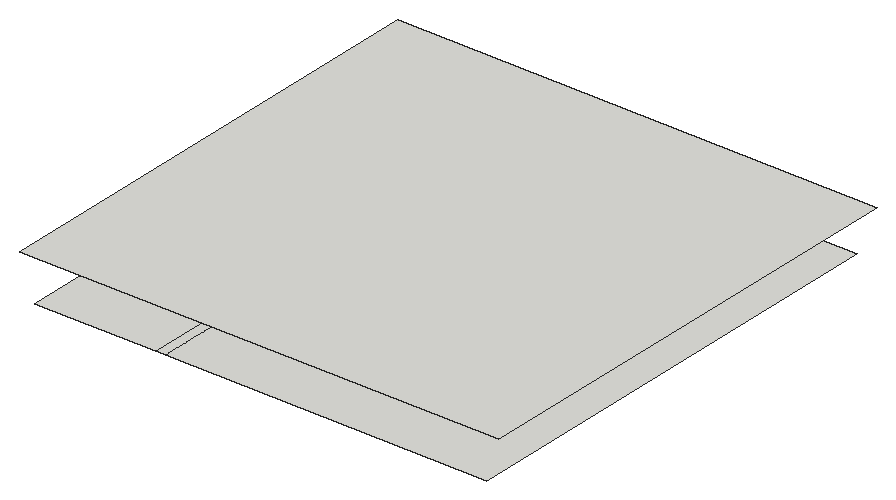
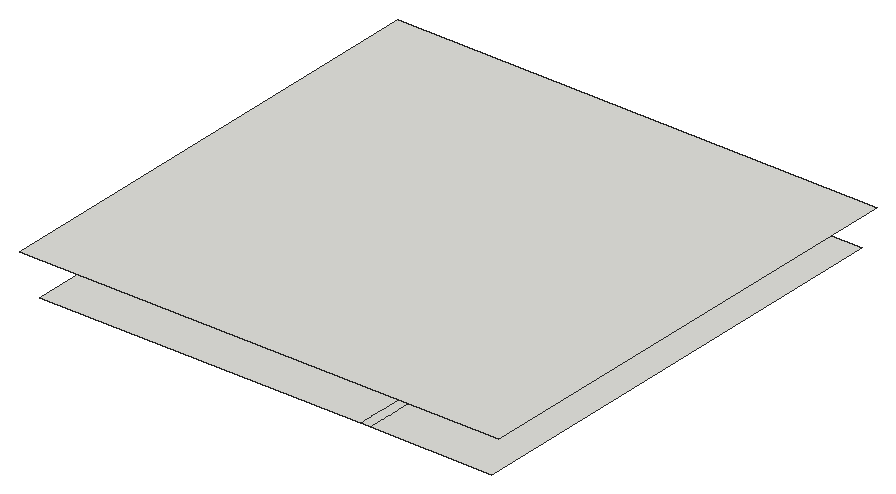
# SketchUp Ruby script. Lengths in inches.
U = 1.inch
M = Sketchup.active_model
def pt(a) = Geom::Point3d.new(a.map { |v| v * U })
def face(e, loops, mat)
  f = e.add_face(loops[0].map { |a| pt(a) })
  loops[1..].each { |l| e.add_face(l.map { |a| pt(a) }).erase! }
  f.material = f.back_material = mat if mat
  f
end
# faces: each face lists its corners as indices into pts; further lists are holes
def faces(e, pts, list, mat = nil) = list.each { |f| face(e, (f[0].is_a?(Array) ? f : [f]).map { |l| l.map { |i| pts[i] } }, mat) }
# xy, xz, yz: faces in a plane at the given z, y or x. An outline is a flat list of corners, or four numbers for a rectangle; further outlines are holes
def ring(l) = l.size == 4 ? [[l[0], l[1]], [l[2], l[1]], [l[2], l[3]], [l[0], l[3]]] : l.each_slice(2).to_a
def flat(e, list, mat, &to3) = list.each { |f| face(e, (f[0].is_a?(Array) ? f : [f]).map { |l| ring(l).map { |u, v| to3.(u, v) } }, mat) }
def xy(e, z, list, mat = nil) = flat(e, list, mat) { |x, y| [x, y, z] }
def xz(e, y, list, mat = nil) = flat(e, list, mat) { |x, z| [x, y, z] }
def yz(e, x, list, mat = nil) = flat(e, list, mat) { |y, z| [x, y, z] }
def lines(e, pts, list) = list.each { |a, b| e.add_line(pt(pts[a]), pt(pts[b])) }
# prism: a flat outline (further loops are holes) pulled along v
def prism(e, loops, v, mat = nil)
  f = face(e, loops, mat); d = Geom::Vector3d.new(v.map { |x| x * U })
  f.pushpull(f.normal.samedirection?(d) ? d.length : -d.length)
end
def box(e, o, s, mat = nil) = prism(e, [[o, [o[0] + s[0], o[1], o[2]], [o[0] + s[0], o[1] + s[1], o[2]], [o[0], o[1] + s[1], o[2]]]], [0, 0, s[2]], mat)
def at(x, y, z, deg = 0) = Geom::Transformation.translation(pt([x, y, z])) * Geom::Transformation.rotation(ORIGIN, Z_AXIS, deg.degrees)
def axes(o, x, y, z) = Geom::Transformation.new([*x, 0, *y, 0, *z, 0, *pt(o).to_a, 1])
def part(name) = M.definitions.add(name)
# library, detail: a bought-in or finely detailed component or shape, given as its bounding box
def library(name, o, s) = part(name).tap { |d| box(d.entities, o, s) }
def detail(e, o, s) = box(e.add_group.entities, o, s)
def put(e, d, t, mat = nil) = e.add_instance(d, t).tap { |i| i.material = mat if mat }
def group(e, t, mat = nil) = e.add_group.tap { |g| g.transformation = t; g.material = mat if mat }.entities
root = M.entities
M.materials.add("[Wood Veneer 01]").color = [120, 70, 37]
xy(root,152.95,[[[101.27,14.42,137.48,92.99],[119.24,38.31,120.375,38.46,121.43,38.89,122.33,39.59,123.03,40.5,123.47,41.55,123.62,42.68,123.47,43.82,123.03,44.87,122.33,45.78,121.43,46.47,120.375,46.91,119.24,47.06,118.11,46.91,117.05,46.47,116.15,45.78,115.45,44.87,115.02,43.82,114.87,42.68,115.02,41.55,115.45,40.5,116.15,39.59,117.05,38.89,118.11,38.46]],[[144.99,14.42,181.2,92.99],[162.74,38.31,163.875,38.46,164.93,38.89,165.83,39.59,166.53,40.5,166.97,41.55,167.12,42.68,166.97,43.82,166.53,44.87,165.83,45.78,164.93,46.47,163.875,46.91,162.74,47.06,161.61,46.91,160.55,46.47,159.65,45.78,158.95,44.87,158.52,43.82,158.37,42.68,158.52,41.55,158.95,40.5,159.65,39.59,160.55,38.89,161.61,38.46]],[[188.72,14.42,224.93,92.99],[207.49,38.31,208.625,38.46,209.68,38.89,210.58,39.59,211.28,40.5,211.72,41.55,211.87,42.68,211.72,43.82,211.28,44.87,210.58,45.78,209.68,46.47,208.625,46.91,207.49,47.06,206.36,46.91,205.3,46.47,204.4,45.78,203.7,44.87,203.27,43.82,203.12,42.68,203.27,41.55,203.7,40.5,204.4,39.59,205.3,38.89,206.36,38.46]],[[232.44,14.42,268.65,92.99],[253.24,38.31,254.375,38.46,255.43,38.89,256.33,39.59,257.03,40.5,257.47,41.55,257.62,42.68,257.47,43.82,257.03,44.87,256.33,45.78,255.43,46.47,254.375,46.91,253.24,47.06,252.11,46.91,251.05,46.47,250.15,45.78,249.45,44.87,249.02,43.82,248.87,42.68,249.02,41.55,249.45,40.5,250.15,39.59,251.05,38.89,252.11,38.46]],[144.74,96.75,226.06,182.83],
  [[101.27,100.5,137.48,179.07],[119.24,133.62,120.375,133.77,121.43,134.21,122.33,134.9,123.03,135.81,123.47,136.86,123.62,138,123.47,139.13,123.03,140.18,122.33,141.09,121.43,141.78,120.375,142.22,119.24,142.37,118.11,142.22,117.05,141.78,116.15,141.09,115.45,140.18,115.02,139.13,114.87,138,115.02,136.86,115.45,135.81,116.15,134.9,117.05,134.21,118.11,133.77]],[[232.44,100.5,268.65,179.07],[250.49,133.62,251.625,133.77,252.68,134.21,253.58,134.9,254.28,135.81,254.72,136.86,254.87,138,254.72,139.13,254.28,140.18,253.58,141.09,252.68,141.78,251.625,142.22,250.49,142.37,249.36,142.22,248.3,141.78,247.4,141.09,246.7,140.18,246.27,139.13,246.12,138,246.27,136.86,246.7,135.81,247.4,134.9,248.3,134.21,249.36,133.77]],[[101.27,186.58,137.48,265.15],[117.68,218.37,118.8125,218.52,119.87,218.96,120.77,219.65,121.47,220.56,121.9,221.61,122.05,222.75,121.9,223.88,121.47,224.93,120.77,225.84,119.87,226.53,118.8125,226.97,117.68,227.12,116.55,226.97,115.49,226.53,114.59,225.84,113.89,224.93,113.45,223.88,113.3,222.75,113.45,221.61,113.89,220.56,114.59,219.65,115.49,218.96,116.55,218.52]],[[144.99,186.58,181.2,265.15],[162.87,218.37,164,218.52,165.05,218.96,165.96,219.65,166.66,220.56,167.09,221.61,167.24,222.75,167.09,223.88,166.66,224.93,165.96,225.84,165.05,226.53,164,226.97,162.87,227.12,161.73,226.97,160.68,226.53,159.77,225.84,159.08,224.93,158.64,223.88,158.49,222.75,158.64,221.61,159.08,220.56,159.77,219.65,160.68,218.96,161.73,218.52]],[[188.72,186.58,224.93,265.15],[204.43,218.37,205.5625,218.52,206.62,218.96,207.52,219.65,208.22,220.56,208.65,221.61,208.8,222.75,208.65,223.88,208.22,224.93,207.52,225.84,206.62,226.53,205.5625,226.97,204.43,227.12,203.3,226.97,202.24,226.53,201.34,225.84,200.64,224.93,200.2,223.88,200.05,222.75,200.2,221.61,200.64,220.56,201.34,219.65,202.24,218.96,203.3,218.52]],
  [[232.44,186.58,268.65,265.15],[250.49,218.37,251.625,218.52,252.68,218.96,253.58,219.65,254.28,220.56,254.72,221.61,254.87,222.75,254.72,223.88,254.28,224.93,253.58,225.84,252.68,226.53,251.625,226.97,250.49,227.12,249.36,226.97,248.3,226.53,247.4,225.84,246.7,224.93,246.27,223.88,246.12,222.75,246.27,221.61,246.7,220.56,247.4,219.65,248.3,218.96,249.36,218.52]]],"[Wood Veneer 01]")
xy(root,154.7,[[119.24,38.31,118.11,38.46,117.05,38.89,116.15,39.59,115.45,40.5,115.02,41.55,114.87,42.68,115.02,43.82,115.45,44.87,116.15,45.78,117.05,46.47,118.11,46.91,119.24,47.06,120.375,46.91,121.43,46.47,122.33,45.78,123.03,44.87,123.47,43.82,123.62,42.68,123.47,41.55,123.03,40.5,122.33,39.59,121.43,38.89,120.375,38.46],[162.74,38.31,161.61,38.46,160.55,38.89,159.65,39.59,158.95,40.5,158.52,41.55,158.37,42.68,158.52,43.82,158.95,44.87,159.65,45.78,160.55,46.47,161.61,46.91,162.74,47.06,163.875,46.91,164.93,46.47,165.83,45.78,166.53,44.87,166.97,43.82,167.12,42.68,166.97,41.55,166.53,40.5,165.83,39.59,164.93,38.89,163.875,38.46],[207.49,38.31,206.36,38.46,205.3,38.89,204.4,39.59,203.7,40.5,203.27,41.55,203.12,42.68,203.27,43.82,203.7,44.87,204.4,45.78,205.3,46.47,206.36,46.91,207.49,47.06,208.625,46.91,209.68,46.47,210.58,45.78,211.28,44.87,211.72,43.82,211.87,42.68,211.72,41.55,211.28,40.5,210.58,39.59,209.68,38.89,208.625,38.46],[253.24,38.31,252.11,38.46,251.05,38.89,250.15,39.59,249.45,40.5,249.02,41.55,248.87,42.68,249.02,43.82,249.45,44.87,250.15,45.78,251.05,46.47,252.11,46.91,253.24,47.06,254.375,46.91,255.43,46.47,256.33,45.78,257.03,44.87,257.47,43.82,257.62,42.68,257.47,41.55,257.03,40.5,256.33,39.59,255.43,38.89,254.375,38.46],[119.24,133.62,118.11,133.77,117.05,134.21,116.15,134.9,115.45,135.81,115.02,136.86,114.87,138,115.02,139.13,115.45,140.18,116.15,141.09,117.05,141.78,118.11,142.22,119.24,142.37,120.375,142.22,121.43,141.78,122.33,141.09,123.03,140.18,123.47,139.13,123.62,138,123.47,136.86,123.03,135.81,122.33,134.9,121.43,134.21,120.375,133.77],
  [250.49,133.62,249.36,133.77,248.3,134.21,247.4,134.9,246.7,135.81,246.27,136.86,246.12,138,246.27,139.13,246.7,140.18,247.4,141.09,248.3,141.78,249.36,142.22,250.49,142.37,251.625,142.22,252.68,141.78,253.58,141.09,254.28,140.18,254.72,139.13,254.87,138,254.72,136.86,254.28,135.81,253.58,134.9,252.68,134.21,251.625,133.77],[117.68,218.37,116.55,218.52,115.49,218.96,114.59,219.65,113.89,220.56,113.45,221.61,113.3,222.75,113.45,223.88,113.89,224.93,114.59,225.84,115.49,226.53,116.55,226.97,117.68,227.12,118.8125,226.97,119.87,226.53,120.77,225.84,121.47,224.93,121.9,223.88,122.05,222.75,121.9,221.61,121.47,220.56,120.77,219.65,119.87,218.96,118.8125,218.52],[162.87,218.37,161.73,218.52,160.68,218.96,159.77,219.65,159.08,220.56,158.64,221.61,158.49,222.75,158.64,223.88,159.08,224.93,159.77,225.84,160.68,226.53,161.73,226.97,162.87,227.12,164,226.97,165.05,226.53,165.96,225.84,166.66,224.93,167.09,223.88,167.24,222.75,167.09,221.61,166.66,220.56,165.96,219.65,165.05,218.96,164,218.52],[204.43,218.37,203.3,218.52,202.24,218.96,201.34,219.65,200.64,220.56,200.2,221.61,200.05,222.75,200.2,223.88,200.64,224.93,201.34,225.84,202.24,226.53,203.3,226.97,204.43,227.12,205.5625,226.97,206.62,226.53,207.52,225.84,208.22,224.93,208.65,223.88,208.8,222.75,208.65,221.61,208.22,220.56,207.52,219.65,206.62,218.96,205.5625,218.52],[250.49,218.37,249.36,218.52,248.3,218.96,247.4,219.65,246.7,220.56,246.27,221.61,246.12,222.75,246.27,223.88,246.7,224.93,247.4,225.84,248.3,226.53,249.36,226.97,250.49,227.12,251.625,226.97,252.68,226.53,253.58,225.84,254.28,224.93,254.72,223.88,254.87,222.75,254.72,221.61,254.28,220.56,253.58,219.65,252.68,218.96,251.625,218.52]])
xy(root,155.0625,[[8.87,0,82.17,279.57],[82.17,0,88.22,279.57],[88.22,0,281.7,279.57]])
xy(root,180.125,[[0,0,289,285.5]])
p = [[119.24,38.31,152.95],[118.11,38.46,152.95],[118.11,38.46,154.7],[119.24,38.31,154.7],[120.375,38.46,152.95],[120.375,38.46,154.7],
  [162.74,38.31,152.95],[161.61,38.46,152.95],[161.61,38.46,154.7],[162.74,38.31,154.7],[163.875,38.46,152.95],[163.875,38.46,154.7],
  [207.49,38.31,152.95],[206.36,38.46,152.95],[206.36,38.46,154.7],[207.49,38.31,154.7],[208.625,38.46,152.95],[208.625,38.46,154.7],
  [253.24,38.31,152.95],[252.11,38.46,152.95],[252.11,38.46,154.7],[253.24,38.31,154.7],[254.375,38.46,152.95],[254.375,38.46,154.7],
  [117.05,38.89,152.95],[117.05,38.89,154.7],[121.43,38.89,152.95],[121.43,38.89,154.7],[160.55,38.89,152.95],[160.55,38.89,154.7],
  [164.93,38.89,152.95],[164.93,38.89,154.7],[205.3,38.89,152.95],[205.3,38.89,154.7],[209.68,38.89,152.95],[209.68,38.89,154.7],
  [251.05,38.89,152.95],[251.05,38.89,154.7],[255.43,38.89,152.95],[255.43,38.89,154.7],[116.15,39.59,152.95],[116.15,39.59,154.7],
  [122.33,39.59,152.95],[122.33,39.59,154.7],[159.65,39.59,152.95],[159.65,39.59,154.7],[165.83,39.59,152.95],[165.83,39.59,154.7],
  [204.4,39.59,152.95],[204.4,39.59,154.7],[210.58,39.59,152.95],[210.58,39.59,154.7],[250.15,39.59,152.95],[250.15,39.59,154.7],
  [256.33,39.59,152.95],[256.33,39.59,154.7],[115.45,40.5,152.95],[115.45,40.5,154.7],[123.03,40.5,152.95],[123.03,40.5,154.7],
  [158.95,40.5,152.95],[158.95,40.5,154.7],[166.53,40.5,152.95],[166.53,40.5,154.7],[203.7,40.5,152.95],[203.7,40.5,154.7],
  [211.28,40.5,152.95],[211.28,40.5,154.7],[249.45,40.5,152.95],[249.45,40.5,154.7],[257.03,40.5,152.95],[257.03,40.5,154.7],
  [115.02,41.55,152.95],[115.02,41.55,154.7],[123.47,41.55,152.95],[123.47,41.55,154.7],[158.52,41.55,152.95],[158.52,41.55,154.7],
  [166.97,41.55,152.95],[166.97,41.55,154.7],[203.27,41.55,152.95],[203.27,41.55,154.7],[211.72,41.55,152.95],[211.72,41.55,154.7],
  [249.02,41.55,152.95],[249.02,41.55,154.7],[257.47,41.55,152.95],[257.47,41.55,154.7],[114.87,42.68,152.95],[114.87,42.68,154.7],
  [123.62,42.68,152.95],[123.62,42.68,154.7],[158.37,42.68,152.95],[158.37,42.68,154.7],[167.12,42.68,152.95],[167.12,42.68,154.7],
  [203.12,42.68,152.95],[203.12,42.68,154.7],[211.87,42.68,152.95],[211.87,42.68,154.7],[248.87,42.68,152.95],[248.87,42.68,154.7],
  [257.62,42.68,152.95],[257.62,42.68,154.7],[115.02,43.82,152.95],[115.02,43.82,154.7],[123.47,43.82,152.95],[123.47,43.82,154.7],
  [158.52,43.82,152.95],[158.52,43.82,154.7],[166.97,43.82,152.95],[166.97,43.82,154.7],[203.27,43.82,152.95],[203.27,43.82,154.7],
  [211.72,43.82,152.95],[211.72,43.82,154.7],[249.02,43.82,152.95],[249.02,43.82,154.7],[257.47,43.82,152.95],[257.47,43.82,154.7],
  [115.45,44.87,152.95],[115.45,44.87,154.7],[123.03,44.87,152.95],[123.03,44.87,154.7],[158.95,44.87,152.95],[158.95,44.87,154.7],
  [166.53,44.87,152.95],[166.53,44.87,154.7],[203.7,44.87,152.95],[203.7,44.87,154.7],[211.28,44.87,152.95],[211.28,44.87,154.7],
  [249.45,44.87,152.95],[249.45,44.87,154.7],[257.03,44.87,152.95],[257.03,44.87,154.7],[116.15,45.78,152.95],[116.15,45.78,154.7],
  [122.33,45.78,152.95],[122.33,45.78,154.7],[159.65,45.78,152.95],[159.65,45.78,154.7],[165.83,45.78,152.95],[165.83,45.78,154.7],
  [204.4,45.78,152.95],[204.4,45.78,154.7],[210.58,45.78,152.95],[210.58,45.78,154.7],[250.15,45.78,152.95],[250.15,45.78,154.7],
  [256.33,45.78,152.95],[256.33,45.78,154.7],[117.05,46.47,152.95],[117.05,46.47,154.7],[121.43,46.47,152.95],[121.43,46.47,154.7],
  [160.55,46.47,152.95],[160.55,46.47,154.7],[164.93,46.47,152.95],[164.93,46.47,154.7],[205.3,46.47,152.95],[205.3,46.47,154.7],
  [209.68,46.47,152.95],[209.68,46.47,154.7],[251.05,46.47,152.95],[251.05,46.47,154.7],[255.43,46.47,152.95],[255.43,46.47,154.7],
  [118.11,46.91,152.95],[118.11,46.91,154.7],[120.375,46.91,152.95],[120.375,46.91,154.7],[161.61,46.91,152.95],[161.61,46.91,154.7],
  [163.875,46.91,152.95],[163.875,46.91,154.7],[206.36,46.91,152.95],[206.36,46.91,154.7],[208.625,46.91,152.95],[208.625,46.91,154.7],
  [252.11,46.91,152.95],[252.11,46.91,154.7],[254.375,46.91,152.95],[254.375,46.91,154.7],[119.24,47.06,152.95],[119.24,47.06,154.7],
  [162.74,47.06,152.95],[162.74,47.06,154.7],[207.49,47.06,152.95],[207.49,47.06,154.7],[253.24,47.06,152.95],[253.24,47.06,154.7],
  [119.24,133.62,152.95],[118.11,133.77,152.95],[118.11,133.77,154.7],[119.24,133.62,154.7],[120.375,133.77,152.95],[120.375,133.77,154.7],
  [250.49,133.62,152.95],[249.36,133.77,152.95],[249.36,133.77,154.7],[250.49,133.62,154.7],[251.625,133.77,152.95],[251.625,133.77,154.7],
  [117.05,134.21,152.95],[117.05,134.21,154.7],[121.43,134.21,152.95],[121.43,134.21,154.7],[248.3,134.21,152.95],[248.3,134.21,154.7],
  [252.68,134.21,152.95],[252.68,134.21,154.7],[116.15,134.9,152.95],[116.15,134.9,154.7],[122.33,134.9,152.95],[122.33,134.9,154.7],
  [247.4,134.9,152.95],[247.4,134.9,154.7],[253.58,134.9,152.95],[253.58,134.9,154.7],[115.45,135.81,152.95],[115.45,135.81,154.7],
  [123.03,135.81,152.95],[123.03,135.81,154.7],[246.7,135.81,152.95],[246.7,135.81,154.7],[254.28,135.81,152.95],[254.28,135.81,154.7],
  [115.02,136.86,152.95],[115.02,136.86,154.7],[123.47,136.86,152.95],[123.47,136.86,154.7],[246.27,136.86,152.95],[246.27,136.86,154.7],
  [254.72,136.86,152.95],[254.72,136.86,154.7],[114.87,138,152.95],[114.87,138,154.7],[123.62,138,152.95],[123.62,138,154.7],
  [246.12,138,152.95],[246.12,138,154.7],[254.87,138,152.95],[254.87,138,154.7],[115.02,139.13,152.95],[115.02,139.13,154.7],
  [123.47,139.13,152.95],[123.47,139.13,154.7],[246.27,139.13,152.95],[246.27,139.13,154.7],[254.72,139.13,152.95],[254.72,139.13,154.7],
  [115.45,140.18,152.95],[115.45,140.18,154.7],[123.03,140.18,152.95],[123.03,140.18,154.7],[246.7,140.18,152.95],[246.7,140.18,154.7],
  [254.28,140.18,152.95],[254.28,140.18,154.7],[116.15,141.09,152.95],[116.15,141.09,154.7],[122.33,141.09,152.95],[122.33,141.09,154.7],
  [247.4,141.09,152.95],[247.4,141.09,154.7],[253.58,141.09,152.95],[253.58,141.09,154.7],[117.05,141.78,152.95],[117.05,141.78,154.7],
  [121.43,141.78,152.95],[121.43,141.78,154.7],[248.3,141.78,152.95],[248.3,141.78,154.7],[252.68,141.78,152.95],[252.68,141.78,154.7],
  [118.11,142.22,152.95],[118.11,142.22,154.7],[120.375,142.22,152.95],[120.375,142.22,154.7],[249.36,142.22,152.95],[249.36,142.22,154.7],
  [251.625,142.22,152.95],[251.625,142.22,154.7],[119.24,142.37,152.95],[119.24,142.37,154.7],[250.49,142.37,152.95],[250.49,142.37,154.7],
  [117.68,218.37,152.95],[116.55,218.52,152.95],[116.55,218.52,154.7],[117.68,218.37,154.7],[118.8125,218.52,152.95],[118.8125,218.52,154.7],
  [162.87,218.37,152.95],[161.73,218.52,152.95],[161.73,218.52,154.7],[162.87,218.37,154.7],[164,218.52,152.95],[164,218.52,154.7],
  [204.43,218.37,152.95],[203.3,218.52,152.95],[203.3,218.52,154.7],[204.43,218.37,154.7],[205.5625,218.52,152.95],[205.5625,218.52,154.7],
  [250.49,218.37,152.95],[249.36,218.52,152.95],[249.36,218.52,154.7],[250.49,218.37,154.7],[251.625,218.52,152.95],[251.625,218.52,154.7],
  [115.49,218.96,152.95],[115.49,218.96,154.7],[119.87,218.96,152.95],[119.87,218.96,154.7],[160.68,218.96,152.95],[160.68,218.96,154.7],
  [165.05,218.96,152.95],[165.05,218.96,154.7],[202.24,218.96,152.95],[202.24,218.96,154.7],[206.62,218.96,152.95],[206.62,218.96,154.7],
  [248.3,218.96,152.95],[248.3,218.96,154.7],[252.68,218.96,152.95],[252.68,218.96,154.7],[114.59,219.65,152.95],[114.59,219.65,154.7],
  [120.77,219.65,152.95],[120.77,219.65,154.7],[159.77,219.65,152.95],[159.77,219.65,154.7],[165.96,219.65,152.95],[165.96,219.65,154.7],
  [201.34,219.65,152.95],[201.34,219.65,154.7],[207.52,219.65,152.95],[207.52,219.65,154.7],[247.4,219.65,152.95],[247.4,219.65,154.7],
  [253.58,219.65,152.95],[253.58,219.65,154.7],[113.89,220.56,152.95],[113.89,220.56,154.7],[121.47,220.56,152.95],[121.47,220.56,154.7],
  [159.08,220.56,152.95],[159.08,220.56,154.7],[166.66,220.56,152.95],[166.66,220.56,154.7],[200.64,220.56,152.95],[200.64,220.56,154.7],
  [208.22,220.56,152.95],[208.22,220.56,154.7],[246.7,220.56,152.95],[246.7,220.56,154.7],[254.28,220.56,152.95],[254.28,220.56,154.7],
  [113.45,221.61,152.95],[113.45,221.61,154.7],[121.9,221.61,152.95],[121.9,221.61,154.7],[158.64,221.61,152.95],[158.64,221.61,154.7],
  [167.09,221.61,152.95],[167.09,221.61,154.7],[200.2,221.61,152.95],[200.2,221.61,154.7],[208.65,221.61,152.95],[208.65,221.61,154.7],
  [246.27,221.61,152.95],[246.27,221.61,154.7],[254.72,221.61,152.95],[254.72,221.61,154.7],[113.3,222.75,152.95],[113.3,222.75,154.7],
  [122.05,222.75,152.95],[122.05,222.75,154.7],[158.49,222.75,152.95],[158.49,222.75,154.7],[167.24,222.75,152.95],[167.24,222.75,154.7],
  [200.05,222.75,152.95],[200.05,222.75,154.7],[208.8,222.75,152.95],[208.8,222.75,154.7],[246.12,222.75,152.95],[246.12,222.75,154.7],
  [254.87,222.75,152.95],[254.87,222.75,154.7],[113.45,223.88,152.95],[113.45,223.88,154.7],[121.9,223.88,152.95],[121.9,223.88,154.7],
  [158.64,223.88,152.95],[158.64,223.88,154.7],[167.09,223.88,152.95],[167.09,223.88,154.7],[200.2,223.88,152.95],[200.2,223.88,154.7],
  [208.65,223.88,152.95],[208.65,223.88,154.7],[246.27,223.88,152.95],[246.27,223.88,154.7],[254.72,223.88,152.95],[254.72,223.88,154.7],
  [113.89,224.93,152.95],[113.89,224.93,154.7],[121.47,224.93,152.95],[121.47,224.93,154.7],[159.08,224.93,152.95],[159.08,224.93,154.7],
  [166.66,224.93,152.95],[166.66,224.93,154.7],[200.64,224.93,152.95],[200.64,224.93,154.7],[208.22,224.93,152.95],[208.22,224.93,154.7],
  [246.7,224.93,152.95],[246.7,224.93,154.7],[254.28,224.93,152.95],[254.28,224.93,154.7],[114.59,225.84,152.95],[114.59,225.84,154.7],
  [120.77,225.84,152.95],[120.77,225.84,154.7],[159.77,225.84,152.95],[159.77,225.84,154.7],[165.96,225.84,152.95],[165.96,225.84,154.7],
  [201.34,225.84,152.95],[201.34,225.84,154.7],[207.52,225.84,152.95],[207.52,225.84,154.7],[247.4,225.84,152.95],[247.4,225.84,154.7],
  [253.58,225.84,152.95],[253.58,225.84,154.7],[115.49,226.53,152.95],[115.49,226.53,154.7],[119.87,226.53,152.95],[119.87,226.53,154.7],
  [160.68,226.53,152.95],[160.68,226.53,154.7],[165.05,226.53,152.95],[165.05,226.53,154.7],[202.24,226.53,152.95],[202.24,226.53,154.7],
  [206.62,226.53,152.95],[206.62,226.53,154.7],[248.3,226.53,152.95],[248.3,226.53,154.7],[252.68,226.53,152.95],[252.68,226.53,154.7],
  [116.55,226.97,152.95],[116.55,226.97,154.7],[118.8125,226.97,152.95],[118.8125,226.97,154.7],[161.73,226.97,152.95],[161.73,226.97,154.7],
  [164,226.97,152.95],[164,226.97,154.7],[203.3,226.97,152.95],[203.3,226.97,154.7],[205.5625,226.97,152.95],[205.5625,226.97,154.7],
  [249.36,226.97,152.95],[249.36,226.97,154.7],[251.625,226.97,152.95],[251.625,226.97,154.7],[117.68,227.12,152.95],[117.68,227.12,154.7],
  [162.87,227.12,152.95],[162.87,227.12,154.7],[204.43,227.12,152.95],[204.43,227.12,154.7],[250.49,227.12,152.95],[250.49,227.12,154.7]]
faces(root,p,[[0,1,2,3],[4,0,3,5],[6,7,8,9],[10,6,9,11],[12,13,14,15],[16,12,15,17],[18,19,20,21],[22,18,21,23],
  [1,24,25,2],[26,4,5,27],[7,28,29,8],[30,10,11,31],[13,32,33,14],[34,16,17,35],[19,36,37,20],[38,22,23,39],
  [24,40,41,25],[42,26,27,43],[28,44,45,29],[46,30,31,47],[32,48,49,33],[50,34,35,51],[36,52,53,37],[54,38,39,55],
  [40,56,57,41],[58,42,43,59],[44,60,61,45],[62,46,47,63],[48,64,65,49],[66,50,51,67],[52,68,69,53],[70,54,55,71],
  [56,72,73,57],[74,58,59,75],[60,76,77,61],[78,62,63,79],[64,80,81,65],[82,66,67,83],[68,84,85,69],[86,70,71,87],
  [72,88,89,73],[90,74,75,91],[76,92,93,77],[94,78,79,95],[80,96,97,81],[98,82,83,99],[84,100,101,85],[102,86,87,103],
  [88,104,105,89],[106,90,91,107],[92,108,109,93],[110,94,95,111],[96,112,113,97],[114,98,99,115],[100,116,117,101],[118,102,103,119],
  [104,120,121,105],[122,106,107,123],[108,124,125,109],[126,110,111,127],[112,128,129,113],[130,114,115,131],[116,132,133,117],[134,118,119,135],
  [120,136,137,121],[138,122,123,139],[124,140,141,125],[142,126,127,143],[128,144,145,129],[146,130,131,147],[132,148,149,133],[150,134,135,151],
  [136,152,153,137],[154,138,139,155],[140,156,157,141],[158,142,143,159],[144,160,161,145],[162,146,147,163],[148,164,165,149],[166,150,151,167],
  [152,168,169,153],[170,154,155,171],[156,172,173,157],[174,158,159,175],[160,176,177,161],[178,162,163,179],[164,180,181,165],[182,166,167,183],
  [168,184,185,169],[184,170,171,185],[172,186,187,173],[186,174,175,187],[176,188,189,177],[188,178,179,189],[180,190,191,181],[190,182,183,191],
  [192,193,194,195],[196,192,195,197],[198,199,200,201],[202,198,201,203],[193,204,205,194],[206,196,197,207],[199,208,209,200],[210,202,203,211],
  [204,212,213,205],[214,206,207,215],[208,216,217,209],[218,210,211,219],[212,220,221,213],[222,214,215,223],[216,224,225,217],[226,218,219,227],
  [220,228,229,221],[230,222,223,231],[224,232,233,225],[234,226,227,235],[228,236,237,229],[238,230,231,239],[232,240,241,233],[242,234,235,243],
  [236,244,245,237],[246,238,239,247],[240,248,249,241],[250,242,243,251],[244,252,253,245],[254,246,247,255],[248,256,257,249],[258,250,251,259],
  [252,260,261,253],[262,254,255,263],[256,264,265,257],[266,258,259,267],[260,268,269,261],[270,262,263,271],[264,272,273,265],[274,266,267,275],
  [268,276,277,269],[278,270,271,279],[272,280,281,273],[282,274,275,283],[276,284,285,277],[284,278,279,285],[280,286,287,281],[286,282,283,287],
  [288,289,290,291],[292,288,291,293],[294,295,296,297],[298,294,297,299],[300,301,302,303],[304,300,303,305],[306,307,308,309],[310,306,309,311],
  [289,312,313,290],[314,292,293,315],[295,316,317,296],[318,298,299,319],[301,320,321,302],[322,304,305,323],[307,324,325,308],[326,310,311,327],
  [312,328,329,313],[330,314,315,331],[316,332,333,317],[334,318,319,335],[320,336,337,321],[338,322,323,339],[324,340,341,325],[342,326,327,343],
  [328,344,345,329],[346,330,331,347],[332,348,349,333],[350,334,335,351],[336,352,353,337],[354,338,339,355],[340,356,357,341],[358,342,343,359],
  [344,360,361,345],[362,346,347,363],[348,364,365,349],[366,350,351,367],[352,368,369,353],[370,354,355,371],[356,372,373,357],[374,358,359,375],
  [360,376,377,361],[378,362,363,379],[364,380,381,365],[382,366,367,383],[368,384,385,369],[386,370,371,387],[372,388,389,373],[390,374,375,391],
  [376,392,393,377],[394,378,379,395],[380,396,397,381],[398,382,383,399],[384,400,401,385],[402,386,387,403],[388,404,405,389],[406,390,391,407],
  [392,408,409,393],[410,394,395,411],[396,412,413,397],[414,398,399,415],[400,416,417,401],[418,402,403,419],[404,420,421,405],[422,406,407,423],
  [408,424,425,409],[426,410,411,427],[412,428,429,413],[430,414,415,431],[416,432,433,417],[434,418,419,435],[420,436,437,421],[438,422,423,439],
  [424,440,441,425],[442,426,427,443],[428,444,445,429],[446,430,431,447],[432,448,449,433],[450,434,435,451],[436,452,453,437],[454,438,439,455],
  [440,456,457,441],[458,442,443,459],[444,460,461,445],[462,446,447,463],[448,464,465,449],[466,450,451,467],[452,468,469,453],[470,454,455,471],
  [456,472,473,457],[472,458,459,473],[460,474,475,461],[474,462,463,475],[464,476,477,465],[476,466,467,477],[468,478,479,469],[478,470,471,479]])
